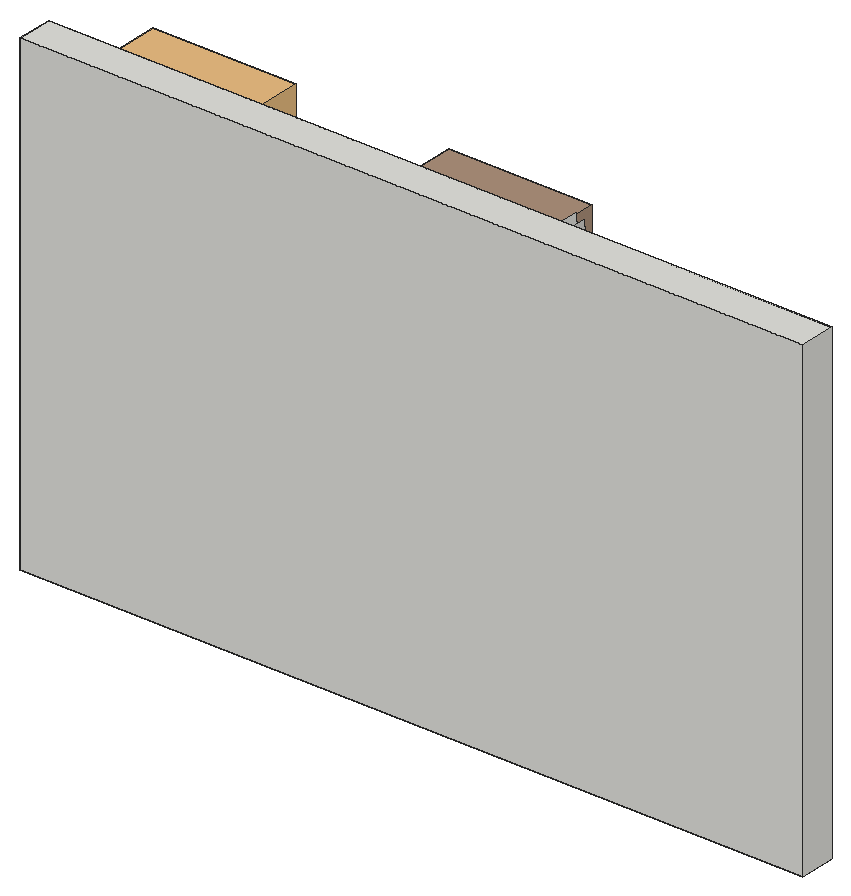
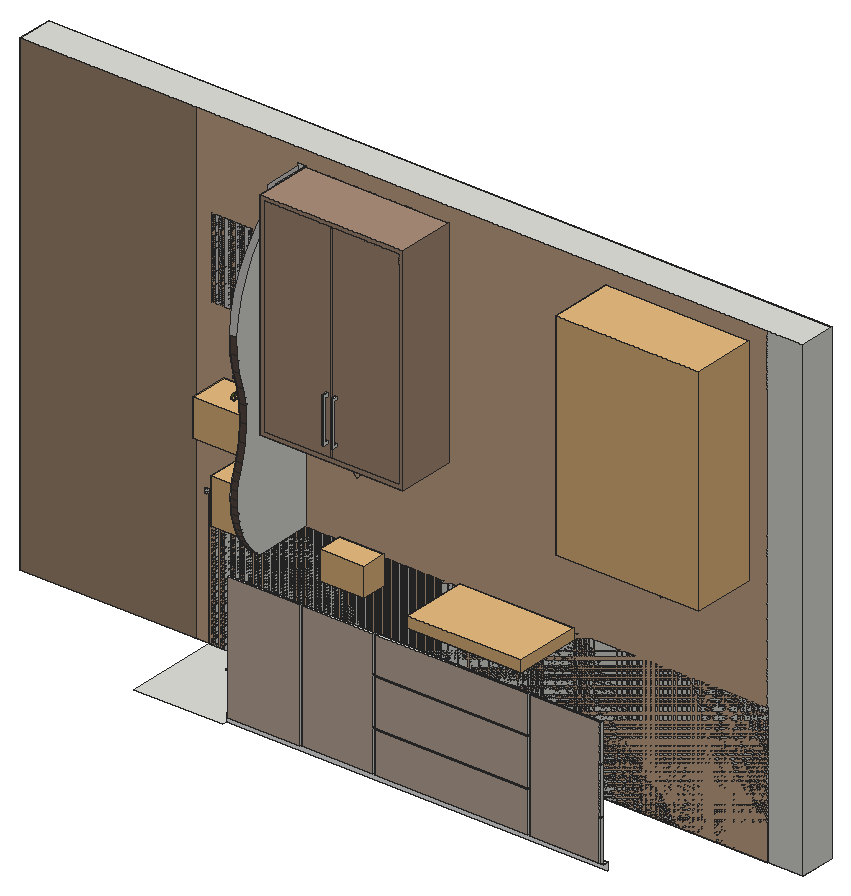
# SketchUp Ruby script. Lengths in inches.
U = 1.inch
M = Sketchup.active_model
def pt(a) = Geom::Point3d.new(a.map { |v| v * U })
def face(e, loops, mat)
  f = e.add_face(loops[0].map { |a| pt(a) })
  loops[1..].each { |l| e.add_face(l.map { |a| pt(a) }).erase! }
  f.material = f.back_material = mat if mat
  f
end
# faces: each face lists its corners as indices into pts; further lists are holes
def faces(e, pts, list, mat = nil) = list.each { |f| face(e, (f[0].is_a?(Array) ? f : [f]).map { |l| l.map { |i| pts[i] } }, mat) }
# xy, xz, yz: faces in a plane at the given z, y or x. An outline is a flat list of corners, or four numbers for a rectangle; further outlines are holes
def ring(l) = l.size == 4 ? [[l[0], l[1]], [l[2], l[1]], [l[2], l[3]], [l[0], l[3]]] : l.each_slice(2).to_a
def flat(e, list, mat, &to3) = list.each { |f| face(e, (f[0].is_a?(Array) ? f : [f]).map { |l| ring(l).map { |u, v| to3.(u, v) } }, mat) }
def xy(e, z, list, mat = nil) = flat(e, list, mat) { |x, y| [x, y, z] }
def xz(e, y, list, mat = nil) = flat(e, list, mat) { |x, z| [x, y, z] }
def yz(e, x, list, mat = nil) = flat(e, list, mat) { |y, z| [x, y, z] }
def lines(e, pts, list) = list.each { |a, b| e.add_line(pt(pts[a]), pt(pts[b])) }
# prism: a flat outline (further loops are holes) pulled along v
def prism(e, loops, v, mat = nil)
  f = face(e, loops, mat); d = Geom::Vector3d.new(v.map { |x| x * U })
  f.pushpull(f.normal.samedirection?(d) ? d.length : -d.length)
end
def box(e, o, s, mat = nil) = prism(e, [[o, [o[0] + s[0], o[1], o[2]], [o[0] + s[0], o[1] + s[1], o[2]], [o[0], o[1] + s[1], o[2]]]], [0, 0, s[2]], mat)
def at(x, y, z, deg = 0) = Geom::Transformation.translation(pt([x, y, z])) * Geom::Transformation.rotation(ORIGIN, Z_AXIS, deg.degrees)
def axes(o, x, y, z) = Geom::Transformation.new([*x, 0, *y, 0, *z, 0, *pt(o).to_a, 1])
def part(name) = M.definitions.add(name)
# library, detail: a bought-in or finely detailed component or shape, given as its bounding box
def library(name, o, s) = part(name).tap { |d| box(d.entities, o, s) }
def detail(e, o, s) = box(e.add_group.entities, o, s)
def put(e, d, t, mat = nil) = e.add_instance(d, t).tap { |i| i.material = mat if mat }
def group(e, t, mat = nil) = e.add_group.tap { |g| g.transformation = t; g.material = mat if mat }.entities
root = M.entities
M.materials.add("2").color = [91, 76, 69]
M.materials.add("Emissive\#2").color = [255, 255, 255]
M.materials.add("Material 3").color = [173, 145, 123]
M.materials.add("[0008_LavenderBlush]").color = [212, 210, 207]
M.materials.add("[Asphalt_New]").color = [85, 106, 44]
M.materials.add("[Color A01]5").color = [206, 173, 143]
M.materials.add("[Color A01]6").color = [165, 139, 115]
M.materials.add("[Color D01]").color = [201, 180, 165]
M.materials.add("white").color = [255, 255, 255]
c1 = part("Component\#59")
xy(c1.entities,0,[[5.79,0,4.75,0.06,3.73,0.22,2.73,0.5,1.77,0.88,0.86,1.37,0,1.95,0.83,2.59,1.74,3.13,2.7,3.56,3.7,3.87,4.74,4.05,5.79,4.12,6.84,4.05,7.87,3.87,8.88,3.56,9.84,3.13,10.74,2.59,11.57,1.95,10.72,1.37,9.8,0.88,8.84,0.5,7.84,0.22,6.82,0.06]],"[Asphalt_New]")
c2 = part("Leaf cluster")
put(c2.entities,c1,axes([10.37,9.23,1.73],[-0.67725,-0.67301,0.29729],[0.61625,-0.73963,-0.27052],[0.40195,0,0.91566]),"[Asphalt_New]")
put(c2.entities,c1,at(0,5.84,1.2),"[Asphalt_New]")
put(c2.entities,c1,axes([11.625,9.72,1.52],[-0.61694,-0.11161,0.77906],[-0.02647,-0.98639,-0.16227],[0.78657,-0.12073,0.60559]),"[Asphalt_New]")
put(c2.entities,c1,axes([13.35,8.05,1.98],[-0.1211,0.99122,-0.05316],[-0.90762,-0.13226,-0.39842],[-0.40195,0,0.91566]),"[Asphalt_New]")
c3 = part("Group338\#1")
p = [[0,0,0],[0,0,-4.36],[-1.91,0,-4.36],[12.46,-1.66,0],[-12.46,-1.66,0],[12.46,1.66,0],
  [12.46,0,0],[-12.46,1.66,0],[1.91,0,-4.36],[-12.46,0,0],[0,0,-7.06]]
lines(c3.entities,p,[[0,1],[1,2],[3,4],[5,6],[7,5],[1,8],[9,0],[0,6],[8,10],[4,9],[6,3],[2,10],
  [9,7]])
c4 = part("Rectangle Light\#1")
put(c4.entities,c3,at(0,0,0))
c5 = library("Group\#654",[0,0,0],[9.47,8.24,11.26])
c6 = library("Group\#162",[0,0,0],[36,15.8125,54.13])
c7 = library("Hanging planter",[0,-5.51,0],[18.9,24.41,17.52])
c8 = library("Gas cooktop",[0,0,0],[16.54,28.74,2.76])
c9 = library("Group\#674",[0,0,0],[11.17,6.3,7.18])
c10 = part("Group\#171")
prism(c10.entities,[[[0,0.37,0],[0,0.37,0.25],[0,0.9375,0.25],[0,0.9375,3.625],[0,0.37,3.625],[0,0.37,3.875],[0,1.01,3.875],[0,1.03,3.875],[0,1.05,3.87],[0,1.07,3.86],[0,1.09,3.85],[0,1.11,3.84],[0,1.125,3.83],[0,1.14,3.81],[0,1.16,3.8],[0,1.17,3.78],[0,1.18,3.76],[0,1.18,3.74],[0,1.1875,3.72],[0,1.1875,0.17],[0,1.1875,0.15],[0,1.18,0.125],[0,1.17,0.11],[0,1.16,0.09],[0,1.15,0.07],[0,1.14,0.05],[0,1.12,0.04],[0,1.1,0.02],[0,1.08,0.01],[0,1.0625,0.01],[0,1.04,0],[0,1.02,0]]],[0.125,0,0])
xy(root,6,[[125.9375,9,125.9375,31.3125,127.25,31.3125,127.25,32.625,149.5625,32.625,149.5625,9]])
xy(root,8,[[31.25,31.3125,49.9375,32],[49.9375,31.3125,50.4375,32],[50.4375,31.3125,88.9375,32],[88.9375,31.3125,89.4375,32],[89.4375,31.3125,107.4375,32],
  [107.4375,31.3125,107.9375,32],[31.25,32,31.9375,32.625],[31.9375,32,49.9375,32.625],[50.4375,32,88.9375,32.625],[89.4375,32,107.4375,32.625]])
xy(root,18.125,[[50.4375,32,88.9375,32.625]])
xy(root,18.625,[[50.4375,32,88.9375,32.625]])
xy(root,30.125,[[50.4375,32,88.9375,32.625]])
xy(root,30.625,[[50.4375,32,88.9375,32.625]])
xy(root,39.75,[[31.9375,32,49.9375,32.625],[50.4375,32,88.9375,32.625],[89.4375,32,107.4375,32.625],[107.9375,32,125.9375,32.625]])
xy(root,41,[[125.3125,9,127.1875,23.51]])
xz(root,9,[[8.9375,6,149.5625,6,149.5625,39.6,150.8125,39.6,150.8125,41,8.9375,41],[125.3125,41,127.1875,122.4375]])
xz(root,9,[[127.1875,83.28,148.875,103.38]],"[0008_LavenderBlush]")
xz(root,31.3125,[[31.25,6,127.25,8]],"Emissive\#2")
xz(root,32,[[31.9375,8,49.9375,18.125],[[49.9375,8,49.9375,39.75,50.4375,39.75,50.4375,30.625,88.9375,30.625,88.9375,39.75,89.4375,39.75,89.4375,30.625,107.4375,30.625,107.4375,30.125,89.4375,30.125,89.4375,18.625,107.4375,18.625,107.4375,18.125,89.4375,18.125,89.4375,8,88.9375,8,88.9375,18.125,50.4375,18.125,50.4375,8],[50.4375,18.625,88.9375,30.125]],[50.4375,8,88.9375,18.125],[89.4375,8,107.4375,18.125],[107.4375,8,107.9375,39.75],
  [31.9375,18.125,49.9375,18.625],[107.9375,18.125,126.5625,18.625],[31.9375,18.625,49.9375,30.125],[50.4375,18.625,88.9375,30.125],[89.4375,18.625,107.4375,30.125],
  [107.9375,18.625,125.9375,30.125],[125.9375,18.625,126.5625,18.75],[31.9375,30.125,49.9375,30.625],[107.9375,30.125,126.5625,30.625],[31.9375,30.625,49.9375,39.75],
  [50.4375,30.625,88.9375,39.75],[89.4375,30.625,107.4375,39.75],[107.9375,30.625,125.9375,39.75]])
xz(root,32.625,[[31.9375,8,32.5625,18.125],[31.9375,18.625,32.5625,30.125],[31.9375,30.625,32.5625,39.75]])
xz(root,32.625,[[32.5625,8,49.9375,39.75],[50.4375,8,88.9375,18.125],[89.4375,8,107.4375,39.75],[107.9375,8,125.9375,39.75],[50.4375,18.625,88.9375,30.125],
  [50.4375,30.625,88.9375,39.75]],"[Color D01]")
yz(root,31.9375,[[32,8,32.625,18.125],[32,18.625,32.625,30.125],[32,30.625,32.625,39.75]])
yz(root,49.9375,[[32,8,32.625,18.125],[32,18.125,32.625,18.625],[32,18.625,32.625,30.125],[32,30.125,32.625,30.625],[32,30.625,32.625,39.75]])
yz(root,50.4375,[[32,8,32.625,18.125],[32,18.625,32.625,30.125],[32,30.625,32.625,39.75]])
yz(root,88.9375,[[32,8,32.625,18.125],[32,18.625,32.625,30.125],[32,30.625,32.625,39.75]])
yz(root,89.4375,[[32,8,32.625,18.125],[32,18.625,32.625,30.125],[32,30.625,32.625,39.75]])
yz(root,107.4375,[[32,8,32.625,39.75]])
yz(root,107.9375,[[32,8,32.625,39.75]])
yz(root,125.3125,[[9,41,9,122.4375,18.35,122.4375,18.37,121.69,18.43,120.95,18.53,120.22,18.6875,119.49,18.89,118.78,19.14,118.08,19.4375,117.39,19.77,116.73,20.16,116.09,20.58,115.48,21.04,114.9,21.54,114.35,23.03,112.8,25.57,109.32,27.63,105.54,29.16,101.52,30.14,97.33,30.54,93.04,30.37,88.74,29.62,84.5,28.3125,80.4,27.59,76.27,27.39,72.08,27.74,67.89,28.61,63.79,29.3,61.8,29.84,59.97,30.2,58.09,30.36,56.18,30.32,54.26,30.09,52.36,29.67,50.49,29.07,48.68,28.28,46.93,27.32,45.27,26.2,43.72,24.92,42.29,23.51,41]])
yz(root,126.5625,[[32,18.625,32.625,18.75]])
yz(root,127.1875,[[9,59.82,28.36,60.22],[9,82.88,29.1,82.88,29.23,83.28,9,83.28],[29.1,82.88,29.23,83.28,29.62,83.28,29.62,82.88]])
yz(root,127.1875,[[9,41,23.51,41,24.92,42.29,26.2,43.72,27.32,45.27,28.28,46.93,29.07,48.68,29.67,50.49,30.09,52.36,30.32,54.26,30.36,56.18,30.2,58.09,29.84,59.97,29.3,61.8,28.61,63.79,27.74,67.89,27.39,72.08,27.59,76.27,28.3125,80.4,29.1,82.88,9,82.88,9,60.22,28.36,60.22,28.36,59.82,9,59.82],[9,83.28,29.23,83.28,29.62,84.5,30.37,88.74,30.54,93.04,30.14,97.33,29.16,101.52,27.63,105.54,25.57,109.32,23.03,112.8,21.54,114.35,21.04,114.9,20.58,115.48,20.16,116.09,19.77,116.73,19.4375,117.39,19.14,118.08,18.89,118.78,18.6875,119.49,18.53,120.22,18.43,120.95,18.37,121.625,9,121.625,9,103.78,24.3,103.78,24.3,103.38,9,103.38]],"[0008_LavenderBlush]")
p = [[125.3125,23.51,41],[125.3125,24.92,42.29],[127.1875,24.92,42.29],[127.1875,23.51,41],[125.3125,26.2,43.72],[127.1875,26.2,43.72],
  [125.3125,27.32,45.27],[127.1875,27.32,45.27],[125.3125,28.28,46.93],[127.1875,28.28,46.93],[125.3125,29.07,48.68],[127.1875,29.07,48.68],
  [125.3125,29.67,50.49],[127.1875,29.67,50.49],[125.3125,30.09,52.36],[127.1875,30.09,52.36],[125.3125,30.32,54.26],[127.1875,30.32,54.26],
  [125.3125,30.36,56.18],[127.1875,30.36,56.18],[125.3125,30.2,58.09],[127.1875,30.2,58.09],[125.3125,29.84,59.97],[127.1875,29.84,59.97],
  [125.3125,29.3,61.8],[127.1875,29.3,61.8],[127.1875,28.61,63.79],[125.3125,28.61,63.79],[125.3125,27.74,67.89],[127.1875,27.74,67.89],
  [125.3125,27.39,72.08],[127.1875,27.39,72.08],[125.3125,27.59,76.27],[127.1875,27.59,76.27],[125.3125,28.3125,80.4],[127.1875,28.3125,80.4],
  [125.3125,29.62,84.5],[127.1875,29.62,84.5],[127.1875,29.23,83.28],[127.1875,29.1,82.88],[125.3125,30.37,88.74],[127.1875,30.37,88.74],
  [125.3125,30.54,93.04],[127.1875,30.54,93.04],[125.9375,32,18.125],[125.9375,32,8],[127.25,31.3125,6],[127.25,30.125,6],
  [126.5625,32,18.125],[126.5625,31.75,18.125],[126.75,32,18.125],[107.11,23.3125,121.04],[107.11,23.3125,69.1],[107.51,23.3125,121.04],
  [107.51,23.3125,69.1]]
faces(root,p,[[0,1,2,3],[1,4,5,2],[4,6,7,5],[6,8,9,7],[8,10,11,9],[10,12,13,11],[12,14,15,13],[14,16,17,15],
  [16,18,19,17],[18,20,21,19],[20,22,23,21],[22,24,25,23],[26,25,24,27],[27,28,29,26],[28,30,31,29],[30,32,33,31],
  [32,34,35,33],[34,36,37,38,39,35],[36,40,41,37],[40,42,43,41]],"2")
lines(root,p,[[44,45],[46,47],[48,49],[48,50],[51,52],[53,54]])
g1 = group(root,at(0,0,6))
xy(g1,0,[[0,0,197.1875,8.67]])
p = [[0,9,0],[162,9,0],[0,8.67,0]]
lines(g1,p,[[0,1],[2,0]])
g2 = group(g1,at(0,0,0))
xy(g2,120,[[0,0,197.1875,9]])
xz(g2,0,[[0,0,197.1875,120]])
xz(g2,9,[[0,0,9,120]])
xz(g2,9,[[9,0,153,120]],"[Color A01]5")
xz(g2,9,[[153,0,197.1875,120]],"[Color A01]6")
yz(g2,0,[[0,0,9,120]])
yz(g2,197.1875,[[0,0,9,120]])
put(root,c1,axes([137.76,14.05,67.85],[-0.15155,-0.00971,-0.00946],[0.01213,-0.13895,-0.07089],[-0.00352,-0.06102,0.16292]),"[Asphalt_New]")
put(root,c1,axes([137.23,14.35,67.63],[-0.15155,-0.00971,-0.00946],[0.01213,-0.13895,-0.07089],[-0.00352,-0.06102,0.16292]),"[Asphalt_New]")
put(root,c2,axes([138.14,14.47,67.59],[-0.10136,0.11337,0],[-0.11337,-0.10136,0],[0,0,0.17792]),"white")
put(root,c2,axes([135.42,13.84,67.67],[0.1271,-0.08349,0],[0.08349,0.1271,0],[0,0,0.17792]),"white")
put(root,c1,axes([136.85,15.16,67.82],[-0.12443,-0.07482,0.0529],[0.06418,-0.13158,-0.04813],[0.05936,-0.01458,0.16292]),"[Asphalt_New]")
put(root,c1,axes([135.92,15,67.55],[-0.09292,-0.02137,0.13861],[0.00305,-0.15002,-0.02887],[0.12035,-0.0127,0.10775]),"[Asphalt_New]")
put(root,c1,axes([134.18,14.33,67.5],[0.1519,0.00716,0],[-0.00716,0.1519,0],[0,0,0.17792]),"[Asphalt_New]")
put(root,c2,axes([136.43,13.01,68.85],[0.12994,0.079,0],[-0.079,0.12994,0],[0,0,0.17792]),"white")
put(root,c2,axes([134.89,14.14,67.46],[0.1271,-0.08349,0],[0.08349,0.1271,0],[0,0,0.17792]),"white")
put(root,c2,axes([138.56,15.26,68],[-0.12016,0.09321,0],[-0.09321,-0.12016,0],[0,0,0.17792]),"white")
put(root,c1,axes([137.05,15.1875,67.78],[-0.09516,0.0059,0.13861],[-0.03969,-0.14471,-0.02887],[0.11178,-0.04636,0.10775]),"[Asphalt_New]")
put(root,c1,axes([137.3125,15.38,67.85],[-0.15155,-0.00971,-0.00946],[0.01213,-0.13895,-0.07089],[-0.00352,-0.06102,0.16292]),"[Asphalt_New]")
put(root,c2,axes([135.57,13.375,68.13],[0.12994,0.079,0],[-0.079,0.12994,0],[0,0,0.17792]),"white")
put(root,c1,axes([135.2,15.04,67.73],[0.14768,-0.03627,0],[0.03627,0.14768,0],[0,0,0.17792]),"[Asphalt_New]")
put(root,c1,axes([135.81,16.02,67.8],[-0.09806,-0.10708,0.0529],[0.09891,-0.10794,-0.04813],[0.06106,0.00288,0.16292]),"[Asphalt_New]")
put(root,c2,axes([138.22,15.57,67.81],[-0.10136,0.11337,0],[-0.11337,-0.10136,0],[0,0,0.17792]),"white")
put(root,c1,axes([137.24,16.19,68.03],[-0.12443,-0.07482,0.0529],[0.06418,-0.13158,-0.04813],[0.05936,-0.01458,0.16292]),"[Asphalt_New]")
put(root,c1,axes([136.19,16.34,67.59],[-0.09806,-0.10708,0.0529],[0.09891,-0.10794,-0.04813],[0.06106,0.00288,0.16292]),"[Asphalt_New]")
put(root,c4,at(30.6,15.5,67.99,180))
put(root,c4,at(107.22,15.5,67.99,180))
put(root,c2,axes([136.86,13.84,68.85],[0.12739,0.08305,0],[-0.08305,0.12739,0],[0,0,0.17792]),"white")
put(root,c2,axes([135.73,17.0625,67.46],[-0.06975,-0.13513,0],[0.13513,-0.06975,0],[0,0,0.17792]),"white")
put(root,c2,axes([135.96,13.875,68.13],[0.12994,0.079,0],[-0.079,0.12994,0],[0,0,0.17792]),"white")
put(root,c1,axes([136.1875,14.76,67.63],[-0.0255,0.1497,-0.00946],[-0.13692,-0.02659,-0.07089],[-0.06106,-0.00288,0.16292]),"[Asphalt_New]")
put(root,c1,axes([135.99,16.11,67.77],[-0.09292,-0.02137,0.13861],[0.00305,-0.15002,-0.02887],[0.12035,-0.0127,0.10775]),"[Asphalt_New]")
put(root,c1,axes([137.36,15.1,68.81],[-0.00408,0.09525,0.13861],[-0.14807,0.02435,-0.02887],[-0.03442,-0.11602,0.10775]),"[Asphalt_New]")
put(root,c5,at(131.79,20.45,41,-90),"white")
put(root,c2,axes([138.6,15.89,67.59],[-0.10136,0.11337,0],[-0.11337,-0.10136,0],[0,0,0.17792]),"white")
put(root,c2,axes([134.98,15.17,67.67],[0.1271,-0.08349,0],[0.08349,0.1271,0],[0,0,0.17792]),"white")
put(root,c1,axes([134.26,15.43,67.71],[0.1519,0.00716,0],[-0.00716,0.1519,0],[0,0,0.17792]),"[Asphalt_New]")
put(root,c1,axes([137.31,15.3,68.84],[-0.08742,0.11593,0.0529],[-0.12415,-0.07758,-0.04813],[-0.0083,-0.06056,0.16292]),"[Asphalt_New]")
put(root,c2,axes([137.2,15.98,67.59],[-0.10136,0.11337,0],[-0.11337,-0.10136,0],[0,0,0.17792]),"white")
put(root,c2,axes([136,14.17,68.13],[0.12739,0.08305,0],[-0.08305,0.12739,0],[0,0,0.17792]),"white")
put(root,c1,axes([136.59,16.76,68.1875],[0.01842,-0.15074,-0.00946],[0.13802,0.02011,-0.07089],[0.06112,0,0.16292]),"[Asphalt_New]")
put(root,c1,axes([137.44,16.22,68],[-0.09516,0.0059,0.13861],[-0.03969,-0.14471,-0.02887],[0.11178,-0.04636,0.10775]),"[Asphalt_New]")
put(root,c1,axes([136.375,16.42,67.55],[-0.09292,-0.02137,0.13861],[0.00305,-0.15002,-0.02887],[0.12035,-0.0127,0.10775]),"[Asphalt_New]")
put(root,c2,axes([136.93,14.44,68.01],[0.07604,0.1317,0],[-0.1317,0.07604,0],[0,0,0.17792]),"white")
put(root,c1,axes([136.5,15.46,68.09],[-0.00408,0.09525,0.13861],[-0.14807,0.02435,-0.02887],[-0.03442,-0.11602,0.10775]),"[Asphalt_New]")
put(root,c1,axes([134.97,16.52,67.55],[-0.09292,-0.02137,0.13861],[0.00305,-0.15002,-0.02887],[0.12035,-0.0127,0.10775]),"[Asphalt_New]")
put(root,c2,axes([138.56,15.76,67.82],[-0.06499,0.13748,0],[-0.13748,-0.06499,0],[0,0,0.17792]),"white")
put(root,c1,axes([134.64,15.75,67.5],[0.1519,0.00716,0],[-0.00716,0.1519,0],[0,0,0.17792]),"[Asphalt_New]")
put(root,c2,axes([137.64,14.58,67.23],[0.07604,0.1317,0],[-0.1317,0.07604,0],[0,0,0.17792]),"white")
g3 = group(root,at(68.41,9,68),"Material 3")
xy(g3,0,[[20.9,0,56.9,14.3125]])
xy(g3,54.13,[[20.9,0,56.9,14.3125]])
xz(g3,0,[[20.9,0,56.9,54.13]])
xz(g3,14.3125,[[[20.9,0,56.9,54.13],[22,1.09,55.81,53.03]],[22,1.09,55.81,53.03]])
yz(g3,20.9,[[0,0,14.3125,54.13]])
yz(g3,56.9,[[0,0,14.3125,54.13]])
put(root,c1,axes([135.58,16.07,67.94],[0.14768,-0.03627,0],[0.03627,0.14768,0],[0,0,0.17792]),"[Asphalt_New]")
put(root,c1,axes([136.45,15.66,68.13],[-0.08742,0.11593,0.0529],[-0.12415,-0.07758,-0.04813],[-0.0083,-0.06056,0.16292]),"[Asphalt_New]")
put(root,c1,axes([136.375,16.875,67.82],[-0.12443,-0.07482,0.0529],[0.06418,-0.13158,-0.04813],[0.05936,-0.01458,0.16292]),"[Asphalt_New]")
put(root,c1,axes([136.04,16.26,67.73],[0.14768,-0.03627,0],[0.03627,0.14768,0],[0,0,0.17792]),"[Asphalt_New]")
put(root,c2,axes([136.37,14.68,68.13],[0.12739,0.08305,0],[-0.08305,0.12739,0],[0,0,0.17792]),"white")
put(root,c1,axes([136.16,17.29,68.04],[-0.02064,-0.15066,0],[0.15066,-0.02064,0],[0,0,0.17792]),"[Asphalt_New]")
put(root,c1,axes([136.89,15.96,68.09],[-0.00408,0.09525,0.13861],[-0.14807,0.02435,-0.02887],[-0.03442,-0.11602,0.10775]),"[Asphalt_New]")
put(root,c1,axes([137.67,16.15,68.84],[-0.09102,0.11312,0.0529],[-0.12166,-0.08144,-0.04813],[-0.00639,-0.06079,0.16292]),"[Asphalt_New]")
put(root,c2,axes([135.8125,18.17,67.67],[-0.06975,-0.13513,0],[0.13513,-0.06975,0],[0,0,0.17792]),"white")
put(root,c1,axes([136.58,16.9,67.78],[-0.09516,0.0059,0.13861],[-0.03969,-0.14471,-0.02887],[0.11178,-0.04636,0.10775]),"[Asphalt_New]")
put(root,c1,axes([136.85,16.16,68.13],[-0.08742,0.11593,0.0529],[-0.12415,-0.07758,-0.04813],[-0.0083,-0.06056,0.16292]),"[Asphalt_New]")
put(root,c1,axes([136.27,15.86,67.85],[-0.0255,0.1497,-0.00946],[-0.13692,-0.02659,-0.07089],[-0.06106,-0.00288,0.16292]),"[Asphalt_New]")
put(root,c1,axes([136.37,17.59,67.59],[-0.09806,-0.10708,0.0529],[0.09891,-0.10794,-0.04813],[0.06106,0.00288,0.16292]),"[Asphalt_New]")
put(root,c1,axes([135.25,17.68,67.59],[-0.09806,-0.10708,0.0529],[0.09891,-0.10794,-0.04813],[0.06106,0.00288,0.16292]),"[Asphalt_New]")
put(root,c1,axes([134.72,16.75,67.73],[0.14768,-0.03627,0],[0.03627,0.14768,0],[0,0,0.17792]),"[Asphalt_New]")
put(root,c1,axes([136.55,17.79,68.04],[-0.02064,-0.15066,0],[0.15066,-0.02064,0],[0,0,0.17792]),"[Asphalt_New]")
put(root,c1,axes([136.86,16.29,68.09],[-0.00707,0.09508,0.13861],[-0.14876,0.01968,-0.02887],[-0.03076,-0.11704,0.10775]),"[Asphalt_New]")
put(root,c6,at(13.59,9,68),"Material 3")
put(root,c7,axes([133.55,21.88,60.22],[0,-0.52438,0],[0.52438,0,0],[0,0,0.52438]),"white")
put(root,c2,axes([136.2,18.48,67.46],[-0.06975,-0.13513,0],[0.13513,-0.06975,0],[0,0,0.17792]),"white")
put(root,c1,axes([136.81,16.49,68.13],[-0.09102,0.11312,0.0529],[-0.12166,-0.08144,-0.04813],[-0.00639,-0.06079,0.16292]),"[Asphalt_New]")
put(root,c1,axes([136.65,16.18,67.63],[-0.0255,0.1497,-0.00946],[-0.13692,-0.02659,-0.07089],[-0.06106,-0.00288,0.16292]),"[Asphalt_New]")
put(root,c2,axes([134.79,18.57,67.46],[-0.06975,-0.13513,0],[0.13513,-0.06975,0],[0,0,0.17792]),"white")
put(root,c2,axes([137.66,17.23,67.59],[-0.10136,0.11337,0],[-0.11337,-0.10136,0],[0,0,0.17792]),"white")
put(root,c1,axes([135.25,16.27,67.63],[-0.0255,0.1497,-0.00946],[-0.13692,-0.02659,-0.07089],[-0.06106,-0.00288,0.16292]),"[Asphalt_New]")
put(root,c1,axes([136.46,18.11,68.04],[-0.0159,-0.15124,0],[0.15124,-0.0159,0],[0,0,0.17792]),"[Asphalt_New]")
put(root,c2,axes([134.66,17.15,68.14],[0.09591,-0.11801,0],[0.11801,0.09591,0],[0,0,0.17792]),"white")
put(root,c1,axes([137.17,17.94,67.82],[-0.12443,-0.07482,0.0529],[0.06418,-0.13158,-0.04813],[0.05936,-0.01458,0.16292]),"[Asphalt_New]")
put(root,c1,axes([136.56,17.67,67.55],[-0.09292,-0.02137,0.13861],[0.00305,-0.15002,-0.02887],[0.12035,-0.0127,0.10775]),"[Asphalt_New]")
put(root,c2,axes([137.68,15.68,68.5],[0.07604,0.1317,0],[-0.1317,0.07604,0],[0,0,0.17792]),"white")
put(root,c1,axes([135.4375,17.76,67.55],[-0.09292,-0.02137,0.13861],[0.00305,-0.15002,-0.02887],[0.12035,-0.0127,0.10775]),"[Asphalt_New]")
put(root,c1,axes([134.82,17,67.5],[0.1519,0.00716,0],[-0.00716,0.1519,0],[0,0,0.17792]),"[Asphalt_New]")
put(root,c1,axes([137.24,16.8,68.09],[-0.00707,0.09508,0.13861],[-0.14876,0.01968,-0.02887],[-0.03076,-0.11704,0.10775]),"[Asphalt_New]")
put(root,c1,axes([135.49,18.24,67.375],[-0.09806,-0.10708,0.0529],[0.09891,-0.10794,-0.04813],[0.06106,0.00288,0.16292]),"[Asphalt_New]")
put(root,c1,axes([136.52,18.26,67.59],[-0.09806,-0.10708,0.0529],[0.09891,-0.10794,-0.04813],[0.06106,0.00288,0.16292]),"[Asphalt_New]")
put(root,c1,axes([137.18,17,68.13],[-0.09102,0.11312,0.0529],[-0.12166,-0.08144,-0.04813],[-0.00639,-0.06079,0.16292]),"[Asphalt_New]")
put(root,c1,axes([136.77,16.59,67.86],[0.01807,0.15078,-0.00946],[-0.13884,0.01339,-0.07089],[-0.05936,0.01458,0.16292]),"[Asphalt_New]")
put(root,c2,axes([137.9,17.79,67.38],[-0.10136,0.11337,0],[-0.11337,-0.10136,0],[0,0,0.17792]),"white")
put(root,c1,axes([137.375,17.97,67.78],[-0.09516,0.0059,0.13861],[-0.03969,-0.14471,-0.02887],[0.11178,-0.04636,0.10775]),"[Asphalt_New]")
put(root,c1,axes([137.5625,18.41,67.61],[-0.12443,-0.07482,0.0529],[0.06418,-0.13158,-0.04813],[0.05936,-0.01458,0.16292]),"[Asphalt_New]")
put(root,c1,axes([136.84,18.62,68.04],[-0.0159,-0.15124,0],[0.15124,-0.0159,0],[0,0,0.17792]),"[Asphalt_New]")
put(root,c1,axes([135.68,18.32,67.34],[-0.09292,-0.02137,0.13861],[0.00305,-0.15002,-0.02887],[0.12035,-0.0127,0.10775]),"[Asphalt_New]")
put(root,c1,axes([135.52,17.81,67.73],[0.14768,-0.03627,0],[0.03627,0.14768,0],[0,0,0.17792]),"[Asphalt_New]")
put(root,c1,axes([136.71,18.35,67.55],[-0.09292,-0.02137,0.13861],[0.00305,-0.15002,-0.02887],[0.12035,-0.0127,0.10775]),"[Asphalt_New]")
put(root,c2,axes([135.83,16.25,67.61],[0.12994,0.079,0],[-0.079,0.12994,0],[0,0,0.17792]),"white")
put(root,c1,axes([133.9375,17.65,67.28],[0.1519,0.00716,0],[-0.00716,0.1519,0],[0,0,0.17792]),"[Asphalt_New]")
put(root,c1,axes([134.97,17.67,67.5],[0.1519,0.00716,0],[-0.00716,0.1519,0],[0,0,0.17792]),"[Asphalt_New]")
put(root,c1,axes([136.83,17.43,67.63],[-0.0255,0.1497,-0.00946],[-0.13692,-0.02659,-0.07089],[-0.06106,-0.00288,0.16292]),"[Asphalt_New]")
put(root,c2,axes([135.26,19.82,67.46],[-0.06975,-0.13513,0],[0.13513,-0.06975,0],[0,0,0.17792]),"white")
put(root,c1,axes([135.71,17.52,67.63],[-0.0255,0.1497,-0.00946],[-0.13692,-0.02659,-0.07089],[-0.06106,-0.00288,0.16292]),"[Asphalt_New]")
put(root,c1,axes([135.91,18.28,67.51],[0.14768,-0.03627,0],[0.03627,0.14768,0],[0,0,0.17792]),"[Asphalt_New]")
put(root,c2,axes([136.17,17.06,67.61],[0.12739,0.08305,0],[-0.08305,0.12739,0],[0,0,0.17792]),"white")
put(root,c1,axes([137.79,18.26,67.82],[-0.08742,0.11593,0.0529],[-0.12415,-0.07758,-0.04813],[-0.0083,-0.06056,0.16292]),"[Asphalt_New]")
put(root,c2,axes([135.5,20.38,67.24],[-0.06975,-0.13513,0],[0.13513,-0.06975,0],[0,0,0.17792]),"white")
put(root,c1,axes([135.95,18.08,67.42],[-0.0255,0.1497,-0.00946],[-0.13692,-0.02659,-0.07089],[-0.06106,-0.00288,0.16292]),"[Asphalt_New]")
put(root,c1,axes([136.98,18.1,67.63],[-0.0255,0.1497,-0.00946],[-0.13692,-0.02659,-0.07089],[-0.06106,-0.00288,0.16292]),"[Asphalt_New]")
put(root,c1,axes([136.77,18.34,67.57],[-0.00408,0.09525,0.13861],[-0.14807,0.02435,-0.02887],[-0.03442,-0.11602,0.10775]),"[Asphalt_New]")
put(root,c1,axes([136.72,18.54,67.61],[-0.08742,0.11593,0.0529],[-0.12415,-0.07758,-0.04813],[-0.0083,-0.06056,0.16292]),"[Asphalt_New]")
put(root,c1,axes([136.42,20.17,67.51],[-0.02064,-0.15066,0],[0.15066,-0.02064,0],[0,0,0.17792]),"[Asphalt_New]")
put(root,c1,axes([137.03,19.17,67.57],[-0.00707,0.09508,0.13861],[-0.14876,0.01968,-0.02887],[-0.03076,-0.11704,0.10775]),"[Asphalt_New]")
put(root,c1,axes([136.98,19.37,67.61],[-0.09102,0.11312,0.0529],[-0.12166,-0.08144,-0.04813],[-0.00639,-0.06079,0.16292]),"[Asphalt_New]")
put(root,c8,at(84.24,11.78,41,90))
put(root,c1,axes([136.63,20.99,67.51],[-0.0159,-0.15124,0],[0.15124,-0.0159,0],[0,0,0.17792]),"[Asphalt_New]")
put(root,c9,at(109.48,24.42,41,-180),"white")
put(root,c10,axes([106.48,22.71,71.96],[-4.5235,0,0],[0,1.64808,0],[0,0,2.94027]))
put(root,c10,axes([108.73,22.71,71.96],[-4.5235,0,0],[0,1.64808,0],[0,0,2.94027]))
